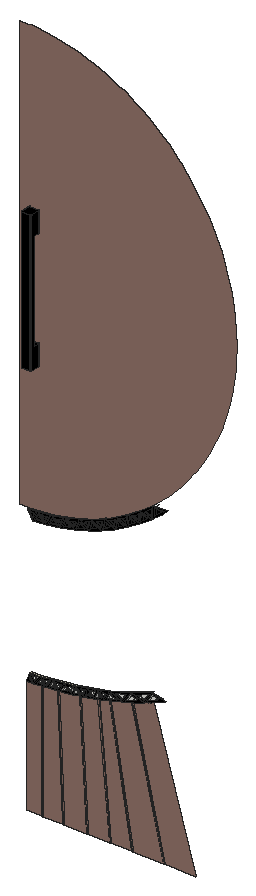
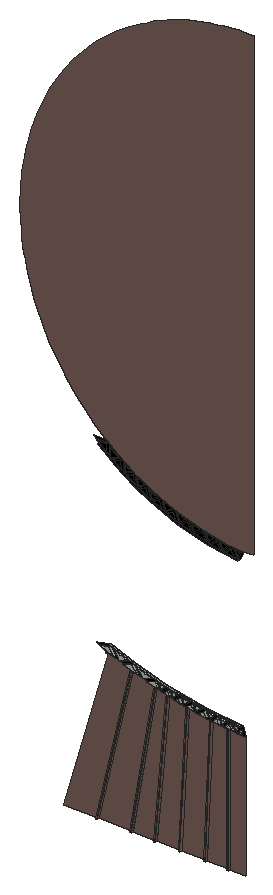
# SketchUp Ruby script. Lengths in inches.
U = 1.inch
M = Sketchup.active_model
def pt(a) = Geom::Point3d.new(a.map { |v| v * U })
def face(e, loops, mat)
  f = e.add_face(loops[0].map { |a| pt(a) })
  loops[1..].each { |l| e.add_face(l.map { |a| pt(a) }).erase! }
  f.material = f.back_material = mat if mat
  f
end
# faces: each face lists its corners as indices into pts; further lists are holes
def faces(e, pts, list, mat = nil) = list.each { |f| face(e, (f[0].is_a?(Array) ? f : [f]).map { |l| l.map { |i| pts[i] } }, mat) }
# xy, xz, yz: faces in a plane at the given z, y or x. An outline is a flat list of corners, or four numbers for a rectangle; further outlines are holes
def ring(l) = l.size == 4 ? [[l[0], l[1]], [l[2], l[1]], [l[2], l[3]], [l[0], l[3]]] : l.each_slice(2).to_a
def flat(e, list, mat, &to3) = list.each { |f| face(e, (f[0].is_a?(Array) ? f : [f]).map { |l| ring(l).map { |u, v| to3.(u, v) } }, mat) }
def xy(e, z, list, mat = nil) = flat(e, list, mat) { |x, y| [x, y, z] }
def xz(e, y, list, mat = nil) = flat(e, list, mat) { |x, z| [x, y, z] }
def yz(e, x, list, mat = nil) = flat(e, list, mat) { |y, z| [x, y, z] }
def lines(e, pts, list) = list.each { |a, b| e.add_line(pt(pts[a]), pt(pts[b])) }
# prism: a flat outline (further loops are holes) pulled along v
def prism(e, loops, v, mat = nil)
  f = face(e, loops, mat); d = Geom::Vector3d.new(v.map { |x| x * U })
  f.pushpull(f.normal.samedirection?(d) ? d.length : -d.length)
end
def box(e, o, s, mat = nil) = prism(e, [[o, [o[0] + s[0], o[1], o[2]], [o[0] + s[0], o[1] + s[1], o[2]], [o[0], o[1] + s[1], o[2]]]], [0, 0, s[2]], mat)
def at(x, y, z, deg = 0) = Geom::Transformation.translation(pt([x, y, z])) * Geom::Transformation.rotation(ORIGIN, Z_AXIS, deg.degrees)
def axes(o, x, y, z) = Geom::Transformation.new([*x, 0, *y, 0, *z, 0, *pt(o).to_a, 1])
def part(name) = M.definitions.add(name)
# library, detail: a bought-in or finely detailed component or shape, given as its bounding box
def library(name, o, s) = part(name).tap { |d| box(d.entities, o, s) }
def detail(e, o, s) = box(e.add_group.entities, o, s)
def put(e, d, t, mat = nil) = e.add_instance(d, t).tap { |i| i.material = mat if mat }
def group(e, t, mat = nil) = e.add_group.tap { |g| g.transformation = t; g.material = mat if mat }.entities
root = M.entities
M.materials.add("Tafisa-Terrarossa-PM780-4K").color = [148, 117, 107]
M.materials.add("Uniboard-L19-Putty-4K").color = [187, 181, 160]
M.materials.add("[Color M09]").color = [0, 0, 0]
xy(root,6.709,[[102.596,138,102.714,138.157],[104.382,138,104.5,138.157],[106.403,138,106.521,138.157],[108.335,138,108.453,138.157],[110.235,138,110.353,138.157]])
xy(root,33.491,[[112.175,138,112.975,138.125]],"[Color M09]")
xz(root,138,[[101.327,6.709,102.596,6.709,102.596,16.558,101.962,16.538,101.327,16.518],[102.714,6.709,104.382,6.709,103.956,16.686,103.581,16.651,103.089,16.604,102.714,16.569],[104.5,6.709,106.403,6.709,105.806,16.94,105.245,16.851,104.567,16.744,104.074,16.697],[106.521,6.709,108.335,6.709,107.371,17.244,107.004,17.162,106.521,17.054,106.222,17.006,105.923,16.959],[108.453,6.709,110.235,6.709,108.339,17.46,107.97,17.377,107.487,17.27],
  [110.353,6.709,112.905,6.709,110.24,18.005,109.403,17.761,108.453,17.485],[113.026,6.709,115.672,6.709,112.104,18.668,111.285,18.373,110.353,18.038]],"Tafisa-Terrarossa-PM780-4K")
xz(root,138,[[[101.327,16.518,101.962,16.538,101.585,17.235],[101.507,16.649,101.608,16.929,101.755,16.657]],[[101.962,16.538,102.552,17.265,101.585,17.235],[101.983,16.762,101.791,17.116,102.282,17.132]],[[101.962,16.538,102.596,16.558,102.714,16.569,103.089,16.604,102.552,17.265],[102.231,16.672,102.552,17.067,102.844,16.707,102.588,16.683]],[[103.089,16.604,103.515,17.356,102.552,17.265],[103.07,16.826,102.796,17.163,103.288,17.209]],[[103.089,16.604,103.581,16.651,103.956,16.686,104.074,16.697,103.515,17.356],[103.316,16.752,103.535,17.139,103.823,16.8,103.57,16.776]],
  [[104.074,16.697,104.478,17.447,103.515,17.356],[104.051,16.918,103.766,17.254,104.257,17.301]],[[104.074,16.697,104.567,16.744,105.245,16.851,104.478,17.447],[104.295,16.844,104.518,17.258,104.94,16.93,104.551,16.868]],[[105.245,16.851,105.433,17.599,104.478,17.447],[105.17,17.068,104.783,17.369,105.265,17.445]],[[105.245,16.851,105.806,16.94,105.923,16.959,106.222,17.006,105.433,17.599],[105.413,17.005,105.509,17.386,105.911,17.084,105.903,17.083]],[[106.222,17.006,106.389,17.75,105.433,17.599],[106.142,17.223,105.745,17.521,106.226,17.598]],
  [[106.222,17.006,106.521,17.054,107.004,17.162,106.389,17.75],[106.385,17.159,106.462,17.506,106.749,17.233,106.498,17.177]],[[107.004,17.162,107.333,17.961,106.389,17.75],[106.958,17.379,106.644,17.679,107.126,17.787]],[[107.004,17.162,107.371,17.244,107.487,17.27,107.97,17.377,107.333,17.961],[107.211,17.336,107.38,17.748,107.708,17.447,107.46,17.392]],[[107.97,17.377,108.277,18.172,107.333,17.961],[107.919,17.594,107.594,17.891,108.076,17.999]],[[107.97,17.377,108.339,17.46,108.453,17.485,109.403,17.761,108.277,18.172],[108.171,17.551,108.349,18.012,109.001,17.775,108.422,17.607]],
  [[109.403,17.761,110.134,18.712,108.277,18.172],[109.36,17.911,108.679,18.159,109.802,18.485]],[[109.403,17.761,110.24,18.005,110.353,18.038,111.285,18.373,110.134,18.712],[109.736,17.988,110.181,18.568,110.882,18.361,110.315,18.157]],[[111.285,18.373,111.955,19.367,110.134,18.712],[111.232,18.519,110.537,18.724,111.637,19.12]],[[111.285,18.373,112.104,18.668,112.216,18.708,113.124,19.101,111.955,19.367],[111.602,18.62,112.011,19.226,112.723,19.064,112.17,18.824]],[[101.823,28.85,102.347,29.707,101.772,29.653,101.422,29.642],[101.833,29.102,101.619,29.525,101.78,29.53,102.114,29.561]],
  [[101.823,28.85,103.023,28.964,102.347,29.707],[102.056,28.996,102.367,29.503,102.766,29.063]],[[103.023,28.964,103.493,29.852,102.922,29.761,102.347,29.707],[102.996,29.176,102.604,29.608,102.9375,29.639,103.269,29.692]],[[103.023,28.964,104.213,29.152,103.493,29.852],[103.247,29.124,103.525,29.649,103.951,29.235]],[[104.213,29.152,104.626,30.068,104.063,29.942,103.493,29.852],[104.173,29.363,103.755,29.769,104.086,29.821,104.413,29.894]],[[104.213,29.152,105.39,29.415,104.626,30.068],[104.427,29.326,104.671,29.868,105.123,29.482]],
  [[105.39,29.415,105.744,30.355,105.19,30.194,104.626,30.068],[105.337,29.623,104.893,30.002,105.221,30.075,105.542,30.168]],[[105.39,29.415,106.547,29.752,105.744,30.355],[105.592,29.602,105.802,30.158,106.277,29.801]],[[106.547,29.752,106.842,30.712,106.299,30.516,105.744,30.355],[106.481,29.955,106.015,30.305,106.337,30.399,106.652,30.513]],[[106.547,29.752,107.682,30.16,106.842,30.712],[106.737,29.951,106.912,30.519,107.408,30.192]],[[107.682,30.16,107.916,31.137,107.386,30.907,106.842,30.712],[107.603,30.359,107.115,30.679,107.431,30.793,107.739,30.926]],
  [[107.682,30.16,108.788,30.639,107.916,31.137],[107.858,30.371,107.997,30.948,108.513,30.654]],[[108.788,30.639,108.96,31.628,108.446,31.366,107.916,31.137],[108.697,30.832,108.19,31.121,108.498,31.255,108.797,31.407]],[[108.788,30.639,109.862,31.186,108.96,31.628],[108.951,30.86,109.053,31.445,109.587,31.184]],[[109.862,31.186,109.972,32.184,109.475,31.89,108.96,31.628],[109.759,31.373,109.235,31.63,109.534,31.782,109.822,31.953]],[[109.862,31.186,110.899,31.799,109.972,32.184],[110.011,31.417,110.076,32.008,110.625,31.78]],
  [[110.899,31.799,110.946,32.803,110.469,32.478,109.972,32.184],[110.785,31.98,110.246,32.204,110.535,32.374,110.812,32.5625]],[[110.899,31.799,111.896,32.477,111.939,32.51,110.946,32.803],[111.034,32.04,111.062,32.64,111.659,32.464]],[[111.939,32.51,112.052,32.598,112.052,33.614,111.424,33.127,110.946,32.803],[111.913,32.646,111.23,32.847,111.496,33.028,111.929,33.363,111.929,32.658]],[[112.052,32.598,112.849,33.216,113.301,33.614,112.052,33.614],[112.175,32.849,112.175,33.491,112.975,33.491,112.77,33.311]]],"[Color M09]")
xz(root,138.125,[[103.247,29.124,103.951,29.235,103.525,29.649],[104.427,29.326,105.123,29.482,104.671,29.868],[104.173,29.363,104.413,29.894,104.086,29.821,103.755,29.769],[105.592,29.602,106.277,29.801,105.802,30.158],[105.337,29.623,105.542,30.168,105.221,30.075,104.893,30.002],
  [106.737,29.951,107.408,30.192,106.912,30.519],[106.481,29.955,106.652,30.513,106.337,30.399,106.015,30.305],[107.603,30.359,107.739,30.926,107.431,30.793,107.115,30.679],[107.858,30.371,108.513,30.654,107.997,30.948],[108.697,30.832,108.797,31.407,108.498,31.255,108.19,31.121],
  [108.951,30.86,109.587,31.184,109.053,31.445],[109.759,31.373,109.822,31.953,109.534,31.782,109.235,31.63],[110.011,31.417,110.625,31.78,110.076,32.008],[110.785,31.98,110.812,32.5625,110.535,32.374,110.246,32.204],[111.034,32.04,111.659,32.464,111.062,32.64],
  [111.913,32.646,111.929,32.658,111.929,33.363,111.496,33.028,111.23,32.847],[112.175,32.849,112.77,33.311,112.975,33.491,112.175,33.491]],"[Color M09]")
xz(root,138.157,[[101.507,16.649,101.755,16.657,101.608,16.929],[102.231,16.672,102.588,16.683,102.844,16.707,102.552,17.067],[103.316,16.752,103.57,16.776,103.823,16.8,103.535,17.139],[101.983,16.762,102.282,17.132,101.791,17.116],[103.07,16.826,103.288,17.209,102.796,17.163],
  [104.295,16.844,104.551,16.868,104.94,16.93,104.518,17.258],[104.051,16.918,104.257,17.301,103.766,17.254],[105.413,17.005,105.903,17.083,105.911,17.084,105.509,17.386],[105.17,17.068,105.265,17.445,104.783,17.369],[106.385,17.159,106.498,17.177,106.749,17.233,106.462,17.506],
  [106.142,17.223,106.226,17.598,105.745,17.521],[107.211,17.336,107.46,17.392,107.708,17.447,107.38,17.748],[106.958,17.379,107.126,17.787,106.644,17.679],[108.171,17.551,108.422,17.607,109.001,17.775,108.349,18.012],[107.919,17.594,108.076,17.999,107.594,17.891],
  [109.36,17.911,109.802,18.485,108.679,18.159],[109.736,17.988,110.315,18.157,110.882,18.361,110.181,18.568],[111.232,18.519,111.637,19.12,110.537,18.724],[111.602,18.62,112.17,18.824,112.723,19.064,112.011,19.226]])
xz(root,138.157,[[102.596,6.709,102.714,6.709,102.714,16.569,102.596,16.558],[104.382,6.709,104.5,6.709,104.074,16.697,103.956,16.686],[106.403,6.709,106.521,6.709,105.923,16.959,105.806,16.94],[108.335,6.709,108.453,6.709,107.487,17.27,107.371,17.244],[110.235,6.709,110.353,6.709,108.453,17.485,108.339,17.46],
  [112.905,6.709,113.026,6.709,110.353,18.038,110.24,18.005],[101.422,29.642,101.772,29.653,102.922,29.761,103.493,29.852,104.063,29.942,104.626,30.068,105.19,30.194,105.744,30.355,106.299,30.516,106.842,30.712,107.386,30.907,107.916,31.137,108.446,31.366,108.96,31.628,109.475,31.89,110.469,32.478,110.946,32.803,111.424,33.127,112.052,33.614,112.336,33.835,113.203,34.599,114.019,35.415,114.331,35.769,114.783,36.282,115.491,37.194,115.509,37.22,116.14,38.15,116.499,38.756,116.728,39.144,117.252,40.173,117.711,41.233,117.906,41.776,118.102,42.319,118.424,43.428,118.676,44.555,118.69,44.641,118.857,45.696,118.911,46.271,118.966,46.846,119.002,48,118.966,49.154,118.857,50.304,118.676,51.445,118.55,52.008,118.424,52.572,118.263,53.126,118.102,53.681,117.711,54.767,117.252,55.827,117.142,56.044,116.728,56.856,116.14,57.85,115.815,58.328,115.491,58.806,114.783,59.718,114.401,60.151,114.019,60.585,113.203,61.401,112.769,61.783,112.336,62.165,111.424,62.873,110.946,63.197,110.469,63.522,109.475,64.11,108.96,64.372,108.446,64.634,107.916,64.863,107.386,65.093,106.842,65.288,106.299,65.484,105.744,65.645,105.19,65.806,104.626,65.932,104.063,66.058,103.493,66.148,102.922,66.239,101.772,66.347,101.597,66.353,101.422,66.358,100.618,66.384,100.618,29.667]],"Tafisa-Terrarossa-PM780-4K")
xz(root,138.157,[[102.056,28.996,102.766,29.063,102.367,29.503],[101.833,29.102,102.114,29.561,101.78,29.53,101.619,29.525],[102.996,29.176,103.269,29.692,102.9375,29.639,102.604,29.608]],"[Color M09]")
yz(root,102.596,[[138,6.709,138.157,16.558]],"Tafisa-Terrarossa-PM780-4K")
yz(root,102.714,[[138,16.558,138.157,16.569]])
yz(root,102.714,[[138,6.709,138.157,16.558]],"Tafisa-Terrarossa-PM780-4K")
yz(root,111.929,[[138,32.658,138.125,33.363]],"[Color M09]")
yz(root,112.175,[[138,32.849,138.125,33.491]],"[Color M09]")
p = [[103.956,138,16.686],[104.382,138,6.709],[104.382,138.157,6.709],[103.956,138.157,16.686],[104.5,138,6.709],[104.074,138,16.697],
  [104.074,138.157,16.697],[104.5,138.157,6.709],[105.806,138,16.94],[106.403,138,6.709],[106.403,138.157,6.709],[105.806,138.157,16.94],
  [106.521,138,6.709],[105.923,138,16.959],[105.923,138.157,16.959],[106.521,138.157,6.709],[107.371,138,17.244],[108.335,138,6.709],
  [108.335,138.157,6.709],[107.371,138.157,17.244],[108.453,138,6.709],[107.487,138,17.27],[107.487,138.157,17.27],[108.453,138.157,6.709],
  [108.339,138,17.46],[110.235,138,6.709],[110.235,138.157,6.709],[108.339,138.157,17.46],[110.353,138,6.709],[108.453,138,17.485],
  [108.453,138.157,17.485],[110.353,138.157,6.709],[110.24,138,18.005],[112.905,138,6.709],[112.905,138.157,6.709],[110.24,138.157,18.005],
  [113.026,138,6.709],[110.353,138,18.038],[110.353,138.157,18.038],[113.026,138.157,6.709],[101.507,138,16.649],[101.755,138,16.657],
  [101.755,138.157,16.657],[101.507,138.157,16.649],[102.714,138,16.569],[102.596,138,16.558],[102.596,138.157,16.558],[102.714,138.157,16.569],
  [101.608,138,16.929],[101.608,138.157,16.929],[102.552,138,17.067],[102.231,138,16.672],[102.231,138.157,16.672],[102.552,138.157,17.067],
  [102.588,138,16.683],[102.588,138.157,16.683],[102.844,138,16.707],[102.844,138.157,16.707],[101.791,138,17.116],[101.983,138,16.762],
  [101.983,138.157,16.762],[101.791,138.157,17.116],[102.282,138,17.132],[102.282,138.157,17.132],[102.796,138,17.163],[103.07,138,16.826],
  [103.07,138.157,16.826],[102.796,138.157,17.163],[103.288,138,17.209],[103.288,138.157,17.209],[103.535,138,17.139],[103.316,138,16.752],
  [103.316,138.157,16.752],[103.535,138.157,17.139],[103.57,138,16.776],[103.57,138.157,16.776],[103.823,138,16.8],[103.823,138.157,16.8],
  [104.518,138,17.258],[104.295,138,16.844],[104.295,138.157,16.844],[104.518,138.157,17.258],[104.551,138,16.868],[104.551,138.157,16.868],
  [103.766,138,17.254],[104.051,138,16.918],[104.051,138.157,16.918],[103.766,138.157,17.254],[104.257,138,17.301],[104.257,138.157,17.301],
  [104.94,138,16.93],[104.94,138.157,16.93],[105.509,138,17.386],[105.413,138,17.005],[105.413,138.157,17.005],[105.509,138.157,17.386],
  [105.903,138,17.083],[105.903,138.157,17.083],[104.783,138,17.369],[105.17,138,17.068],[105.17,138.157,17.068],[104.783,138.157,17.369],
  [105.265,138,17.445],[105.265,138.157,17.445],[105.911,138,17.084],[105.911,138.157,17.084],[101.585,138,17.235],[102.552,138,17.265],
  [102.552,138.157,17.265],[101.585,138.157,17.235],[105.745,138,17.521],[106.142,138,17.223],[106.142,138.157,17.223],[105.745,138.157,17.521],
  [106.226,138,17.598],[106.226,138.157,17.598],[106.462,138,17.506],[106.385,138,17.159],[106.385,138.157,17.159],[106.462,138.157,17.506],
  [106.498,138,17.177],[106.498,138.157,17.177],[106.749,138,17.233],[106.749,138.157,17.233],[103.515,138,17.356],[103.515,138.157,17.356],
  [107.38,138,17.748],[107.211,138,17.336],[107.211,138.157,17.336],[107.38,138.157,17.748],[107.46,138,17.392],[107.46,138.157,17.392],
  [104.478,138,17.447],[104.478,138.157,17.447],[105.433,138,17.599],[105.433,138.157,17.599],[106.644,138,17.679],[106.958,138,17.379],
  [106.958,138.157,17.379],[106.644,138.157,17.679],[107.126,138,17.787],[107.126,138.157,17.787],[107.708,138,17.447],[107.708,138.157,17.447],
  [106.389,138,17.75],[106.389,138.157,17.75],[107.594,138,17.891],[107.919,138,17.594],[107.919,138.157,17.594],[107.594,138.157,17.891],
  [108.076,138,17.999],[108.076,138.157,17.999],[108.349,138,18.012],[108.171,138,17.551],[108.171,138.157,17.551],[108.349,138.157,18.012],
  [108.422,138,17.607],[108.422,138.157,17.607],[109.001,138,17.775],[109.001,138.157,17.775],[107.333,138,17.961],[107.333,138.157,17.961],
  [108.679,138,18.159],[109.36,138,17.911],[109.36,138.157,17.911],[108.679,138.157,18.159],[109.802,138,18.485],[109.802,138.157,18.485],
  [108.277,138,18.172],[108.277,138.157,18.172],[110.181,138,18.568],[109.736,138,17.988],[109.736,138.157,17.988],[110.181,138.157,18.568],
  [110.315,138,18.157],[110.315,138.157,18.157],[110.134,138,18.712],[110.134,138.157,18.712],[110.882,138,18.361],[110.882,138.157,18.361],
  [110.537,138,18.724],[111.232,138,18.519],[111.232,138.157,18.519],[110.537,138.157,18.724],[111.637,138,19.12],[111.637,138.157,19.12],
  [112.011,138,19.226],[111.602,138,18.62],[111.602,138.157,18.62],[112.011,138.157,19.226],[112.17,138,18.824],[112.17,138.157,18.824],
  [111.955,138,19.367],[111.955,138.157,19.367],[112.216,138,18.708],[112.104,138,18.668],[112.104,138.157,18.668],[112.216,138.157,18.708],
  [112.723,138,19.064],[112.723,138.157,19.064],[103.023,138,28.964],[101.823,138,28.85],[101.823,138.157,28.85],[103.023,138.157,28.964],
  [102.367,138,29.503],[102.056,138,28.996],[102.056,138.157,28.996],[102.367,138.157,29.503],[102.766,138,29.063],[102.766,138.157,29.063],
  [104.213,138,29.152],[104.213,138.157,29.152],[101.619,138,29.525],[101.833,138,29.102],[101.833,138.157,29.102],[101.619,138.157,29.525],
  [102.114,138,29.561],[102.114,138.157,29.561],[103.525,138,29.649],[103.247,138,29.124],[103.247,138.125,29.124],[103.525,138.125,29.649],
  [103.951,138,29.235],[103.951,138.125,29.235],[102.604,138,29.608],[102.996,138,29.176],[102.996,138.157,29.176],[102.604,138.157,29.608],
  [103.269,138,29.692],[103.269,138.157,29.692],[105.39,138,29.415],[105.39,138.157,29.415],[104.671,138,29.868],[104.427,138,29.326],
  [104.427,138.125,29.326],[104.671,138.125,29.868],[105.123,138,29.482],[105.123,138.125,29.482],[103.755,138,29.769],[104.173,138,29.363],
  [104.173,138.125,29.363],[103.755,138.125,29.769],[104.413,138,29.894],[104.413,138.125,29.894],[106.547,138,29.752],[106.547,138.157,29.752],
  [101.78,138,29.53],[101.78,138.157,29.53],[101.422,138,29.642],[101.772,138,29.653],[101.772,138.157,29.653],[101.422,138.157,29.642],
  [102.9375,138,29.639],[102.9375,138.157,29.639],[104.893,138,30.002],[105.337,138,29.623],[105.337,138.125,29.623],[104.893,138.125,30.002],
  [105.542,138,30.168],[105.542,138.125,30.168],[105.802,138,30.158],[105.592,138,29.602],[105.592,138.125,29.602],[105.802,138.125,30.158],
  [106.277,138,29.801],[106.277,138.125,29.801],[102.347,138,29.707],[102.347,138.157,29.707],[102.922,138,29.761],[102.922,138.157,29.761],
  [103.493,138,29.852],[103.493,138.157,29.852],[104.086,138,29.821],[104.086,138.125,29.821],[107.682,138,30.16],[107.682,138.157,30.16],
  [104.063,138,29.942],[104.063,138.157,29.942],[104.626,138,30.068],[104.626,138.157,30.068],[105.221,138,30.075],[105.221,138.125,30.075],
  [106.015,138,30.305],[106.481,138,29.955],[106.481,138.125,29.955],[106.015,138.125,30.305],[106.652,138,30.513],[106.652,138.125,30.513],
  [106.912,138,30.519],[106.737,138,29.951],[106.737,138.125,29.951],[106.912,138.125,30.519],[107.408,138,30.192],[107.408,138.125,30.192],
  [105.19,138,30.194],[105.19,138.157,30.194],[105.744,138,30.355],[105.744,138.157,30.355],[108.788,138,30.639],[108.788,138.157,30.639],
  [106.337,138,30.399],[106.337,138.125,30.399],[106.299,138,30.516],[106.299,138.157,30.516],[107.115,138,30.679],[107.603,138,30.359],
  [107.603,138.125,30.359],[107.115,138.125,30.679],[107.739,138,30.926],[107.739,138.125,30.926],[107.997,138,30.948],[107.858,138,30.371],
  [107.858,138.125,30.371],[107.997,138.125,30.948],[108.513,138,30.654],[108.513,138.125,30.654],[106.842,138,30.712],[106.842,138.157,30.712],
  [109.862,138,31.186],[109.862,138.157,31.186],[107.386,138,30.907],[107.386,138.157,30.907],[107.431,138,30.793],[107.431,138.125,30.793],
  [108.19,138,31.121],[108.697,138,30.832],[108.697,138.125,30.832],[108.19,138.125,31.121],[108.797,138,31.407],[108.797,138.125,31.407],
  [107.916,138,31.137],[107.916,138.157,31.137],[109.053,138,31.445],[108.951,138,30.86],[108.951,138.125,30.86],[109.053,138.125,31.445],
  [109.587,138,31.184],[109.587,138.125,31.184],[108.446,138,31.366],[108.446,138.157,31.366],[108.498,138,31.255],[108.498,138.125,31.255],
  [110.899,138,31.799],[110.899,138.157,31.799],[108.96,138,31.628],[108.96,138.157,31.628],[109.235,138,31.63],[109.759,138,31.373],
  [109.759,138.125,31.373],[109.235,138.125,31.63],[109.822,138,31.953],[109.822,138.125,31.953],[110.076,138,32.008],[110.011,138,31.417],
  [110.011,138.125,31.417],[110.076,138.125,32.008],[110.625,138,31.78],[110.625,138.125,31.78],[109.475,138,31.89],[109.475,138.157,31.89],
  [109.534,138,31.782],[109.534,138.125,31.782],[111.896,138,32.477],[111.896,138.157,32.477],[109.972,138,32.184],[109.972,138.157,32.184],
  [110.246,138,32.204],[110.785,138,31.98],[110.785,138.125,31.98],[110.246,138.125,32.204],[110.812,138,32.5625],[110.812,138.125,32.5625],
  [111.062,138,32.64],[111.034,138,32.04],[111.034,138.125,32.04],[111.062,138.125,32.64],[111.659,138,32.464],[111.659,138.125,32.464],
  [110.469,138,32.478],[110.469,138.157,32.478],[110.535,138,32.374],[110.535,138.125,32.374],[110.946,138,32.803],[110.946,138.157,32.803],
  [111.939,138,32.51],[111.939,138.157,32.51],[112.052,138,32.598],[112.052,138.157,32.598],[111.23,138,32.847],[111.913,138,32.646],
  [111.913,138.125,32.646],[111.23,138.125,32.847],[111.929,138,32.658],[111.929,138.125,32.658],[112.849,138,33.216],[112.849,138.157,33.216],
  [111.424,138,33.127],[111.424,138.157,33.127],[111.496,138,33.028],[111.496,138.125,33.028],[112.175,138,32.849],[112.77,138,33.311],
  [112.77,138.125,33.311],[112.175,138.125,32.849],[111.929,138,33.363],[111.929,138.125,33.363],[112.052,138,33.614],[112.052,138.157,33.614],
  [112.336,138,33.835],[112.336,138.157,33.835],[112.415,138,33.74],[112.411,138,33.737],[112.411,138.125,33.737],[112.415,138.125,33.74],
  [112.102,138,18.674],[110.239,138,18.01],[108.335,138,17.485],[107.369,138,17.27],[105.805,138,16.959],[103.956,138,16.697]]
faces(root,p,[[0,1,2,3],[4,5,6,7],[8,9,10,11],[12,13,14,15],[16,17,18,19],[20,21,22,23],[24,25,26,27],[28,29,30,31],
  [32,33,34,35],[36,37,38,39]],"Tafisa-Terrarossa-PM780-4K")
faces(root,p,[[40,41,42,43],[44,45,46,47],[41,48,49,42],[50,51,52,53],[51,54,55,52],[56,50,53,57],[54,56,57,55],[5,0,3,6],
  [58,59,60,61],[59,62,63,60],[64,65,66,67],[65,68,69,66],[70,71,72,73],[71,74,75,72],[76,70,73,77],[74,76,77,75],
  [78,79,80,81],[79,82,83,80],[84,85,86,87],[85,88,89,86],[90,78,81,91],[82,90,91,83],[13,8,11,14],[92,93,94,95],
  [93,96,97,94],[62,58,61,63],[98,99,100,101],[99,102,103,100],[104,92,95,105],[96,104,105,97],[68,64,67,69],[110,111,112,113],
  [111,114,115,112],[116,117,118,119],[117,120,121,118],[122,116,119,123],[120,122,123,121],[21,16,19,22],[88,84,87,89],[126,127,128,129],
  [127,130,131,128],[102,98,101,103],[136,137,138,139],[137,140,141,138],[142,126,129,143],[130,142,143,131],[114,110,113,115],[29,24,27,30],
  [146,147,148,149],[147,150,151,148],[152,153,154,155],[153,156,157,154],[156,158,159,157],[140,136,139,141],[158,152,155,159],[150,146,149,151],
  [162,163,164,165],[163,166,167,164],[170,171,172,173],[171,174,175,172],[37,32,35,38],[166,162,165,167],[174,178,179,175],[178,170,173,179],
  [180,181,182,183],[181,184,185,182],[186,187,188,189],[187,190,191,188],[184,180,183,185],[194,195,196,197],[190,198,199,191],[198,186,189,199]])
faces(root,p,[[106,107,108,109],[107,124,125,108],[124,132,133,125],[132,134,135,133],[134,144,145,135],[144,160,161,145],[160,168,169,161],[168,176,177,169],
  [176,192,193,177]],"Uniboard-L19-Putty-4K")
faces(root,p,[[200,201,202,203],[204,205,206,207],[205,208,209,206],[210,200,203,211],[212,213,214,215],[213,216,217,214],[208,204,207,209],[218,219,220,221],
  [219,222,223,220],[224,225,226,227],[225,228,229,226],[222,218,221,223],[230,210,211,231],[232,233,234,235],[233,236,237,234],[238,239,240,241],
  [239,242,243,240],[244,230,231,245],[246,212,215,247],[216,246,247,217],[236,232,235,237],[248,249,250,251],[252,224,227,253],[228,252,253,229],
  [254,255,256,257],[255,258,259,256],[260,261,262,263],[261,264,265,262],[249,266,267,250],[266,268,269,267],[268,270,271,269],[272,238,241,273],
  [242,272,273,243],[264,260,263,265],[274,244,245,275],[270,276,277,271],[276,278,279,277],[280,254,257,281],[282,283,284,285],[283,286,287,284],
  [288,289,290,291],[289,292,293,290],[278,294,295,279],[258,280,281,259],[294,296,297,295],[292,288,291,293],[298,274,275,299],[300,282,285,301],
  [296,302,303,297],[286,300,301,287],[304,305,306,307],[305,308,309,306],[310,311,312,313],[311,314,315,312],[302,316,317,303],[318,298,299,319],
  [316,320,321,317],[322,304,307,323],[314,310,313,315],[308,322,323,309],[324,325,326,327],[325,328,329,326],[320,330,331,321],[332,333,334,335],
  [333,336,337,334],[330,338,339,331],[340,324,327,341],[336,332,335,337],[342,318,319,343],[328,340,341,329],[338,344,345,339],[346,347,348,349],
  [347,350,351,348],[352,353,354,355],[353,356,357,354],[344,358,359,345],[360,346,349,361],[350,360,361,351],[356,352,355,357],[362,342,343,363],
  [358,364,365,359],[366,367,368,369],[367,370,371,368],[372,373,374,375],[373,376,377,374],[364,378,379,365],[380,366,369,381],[370,380,381,371],
  [378,382,383,379],[376,372,375,377],[384,362,363,385],[386,384,385,387],[388,389,390,391],[389,392,393,390],[394,386,387,395],[382,396,397,383],
  [398,388,391,399],[400,401,402,403],[404,398,399,405],[396,406,407,397],[406,408,409,407],[410,411,412,413]],"[Color M09]")
lines(root,p,[[414,195],[415,32],[416,24],[417,16],[418,8],[419,0]])
g1 = group(root,at(101.59,137.06,52.7))
xy(g1,-11.84,[[0.09,0,0.04,0.01,0.01,0.04,0,0.09,0,0.77,0.01,0.8125,0.04,0.85,0.09,0.86,0.77,0.86,0.8125,0.85,0.85,0.8125,0.86,0.77,0.86,0.09,0.85,0.04,0.81,0.01,0.77,0]],"[Color M09]")
xy(g1,-10.1,[[0,0.45,0.86,0.45,0.86,0.77,0.85,0.8125,0.8125,0.85,0.77,0.86,0.09,0.86,0.04,0.85,0.01,0.8125,0,0.77]],"[Color M09]")
xy(g1,-1.72,[[0,0.45,0,0.77,0.01,0.8125,0.04,0.85,0.09,0.86,0.77,0.86,0.8125,0.85,0.85,0.8125,0.86,0.77,0.86,0.45]],"[Color M09]")
xy(g1,0.02,[[0.09,0,0.77,0,0.81,0.01,0.85,0.04,0.86,0.09,0.86,0.77,0.85,0.8125,0.8125,0.85,0.77,0.86,0.09,0.86,0.04,0.85,0.01,0.8125,0,0.77,0,0.09,0.01,0.04,0.04,0.01]],"[Color M09]")
xz(g1,0,[[0.09,-11.84,0.77,0.02]],"[Color M09]")
xz(g1,0.26,[[0,-9.91,0.86,-1.91]],"[Color M09]")
xz(g1,0.86,[[0.09,-11.84,0.77,-10.1],[0.09,-1.72,0.77,0.02]],"[Color M09]")
yz(g1,0,[[0.09,-11.84,0.09,0.02,0.77,0.02,0.77,-1.72,0.45,-1.72,0.36,-1.75,0.29,-1.82,0.26,-1.91,0.26,-9.91,0.29,-10.01,0.36,-10.07,0.45,-10.1,0.77,-10.1,0.77,-11.84]],"[Color M09]")
yz(g1,0.86,[[0.09,-11.84,0.77,-11.84,0.77,-10.1,0.45,-10.1,0.36,-10.07,0.29,-10.01,0.26,-9.91,0.26,-1.91,0.29,-1.82,0.36,-1.75,0.45,-1.72,0.77,-1.72,0.77,0.02,0.09,0.02]],"[Color M09]")
p = [[0.04,0.01,-11.84],[0.09,0,-11.84],[0.09,0,0.02],[0.04,0.01,0.02],[0.01,0.04,-11.84],[0.01,0.04,0.02],
  [0,0.09,0.02],[0,0.09,-11.84],[0.85,0.04,-11.84],[0.85,0.04,0.02],[0.81,0.01,0.02],[0.81,0.01,-11.84],
  [0.77,0,-11.84],[0.77,0,0.02],[0.86,0.09,-11.84],[0.86,0.09,0.02],[0.01,0.8125,-11.84],[0,0.77,-11.84],
  [0,0.77,-10.1],[0.01,0.8125,-10.1],[0.04,0.85,-11.84],[0.04,0.85,-10.1],[0.09,0.86,-11.84],[0.09,0.86,-10.1],
  [0.8125,0.85,-11.84],[0.77,0.86,-11.84],[0.77,0.86,-10.1],[0.8125,0.85,-10.1],[0.85,0.8125,-11.84],[0.85,0.8125,-10.1],
  [0.86,0.77,-11.84],[0.86,0.77,-10.1],[0.86,0.29,-10.01],[0.86,0.36,-10.07],[0,0.36,-10.07],[0,0.29,-10.01],
  [0.86,0.45,-10.1],[0,0.45,-10.1],[0.86,0.26,-9.91],[0,0.26,-9.91],[0,0.29,-1.82],[0.86,0.29,-1.82],
  [0.86,0.26,-1.91],[0,0.26,-1.91],[0.86,0.36,-1.75],[0,0.36,-1.75],[0.86,0.45,-1.72],[0,0.45,-1.72],
  [0,0.77,-1.72],[0,0.77,0.02],[0.01,0.8125,0.02],[0.01,0.8125,-1.72],[0.04,0.85,0.02],[0.09,0.86,0.02],
  [0.09,0.86,-1.72],[0.04,0.85,-1.72],[0.77,0.86,0.02],[0.8125,0.85,0.02],[0.8125,0.85,-1.72],[0.77,0.86,-1.72],
  [0.85,0.8125,-1.72],[0.85,0.8125,0.02],[0.86,0.77,0.02],[0.86,0.77,-1.72]]
faces(g1,p,[[0,1,2,3],[4,0,3,5],[4,5,6,7],[8,9,10,11],[12,11,10,13],[14,15,9,8],[16,17,18,19],[20,16,19,21],
  [22,20,21,23],[24,25,26,27],[28,24,27,29],[30,28,29,31],[32,33,34,35],[33,36,37,34],[38,32,35,39],[40,41,42,43],
  [44,41,40,45],[46,44,45,47],[48,49,50,51],[52,53,54,55],[51,50,52,55],[56,57,58,59],[60,61,62,63],[57,61,60,58]],"[Color M09]")
